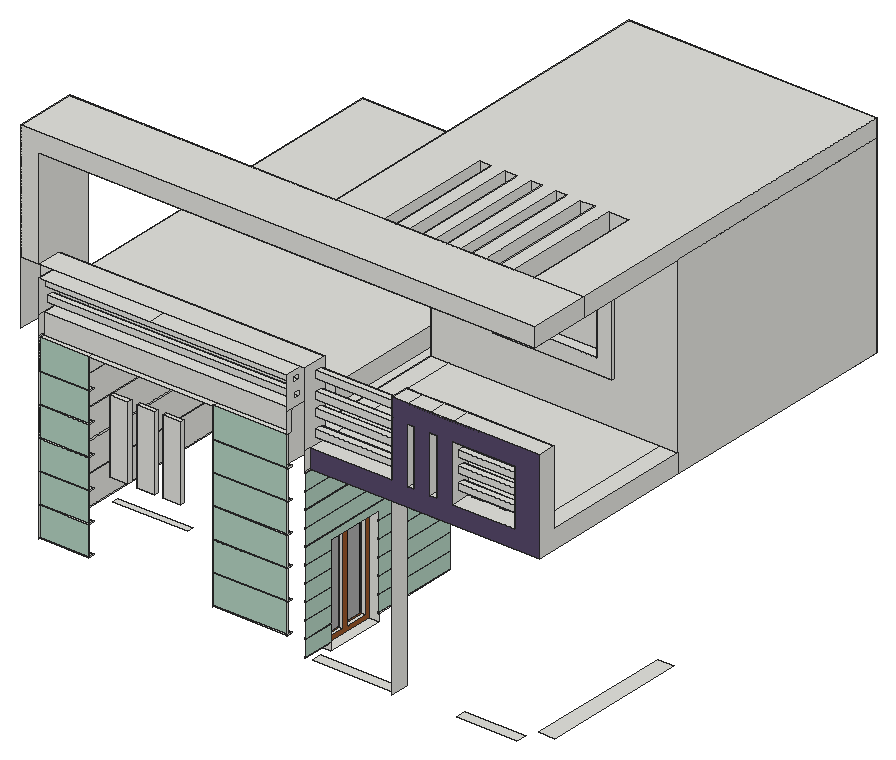
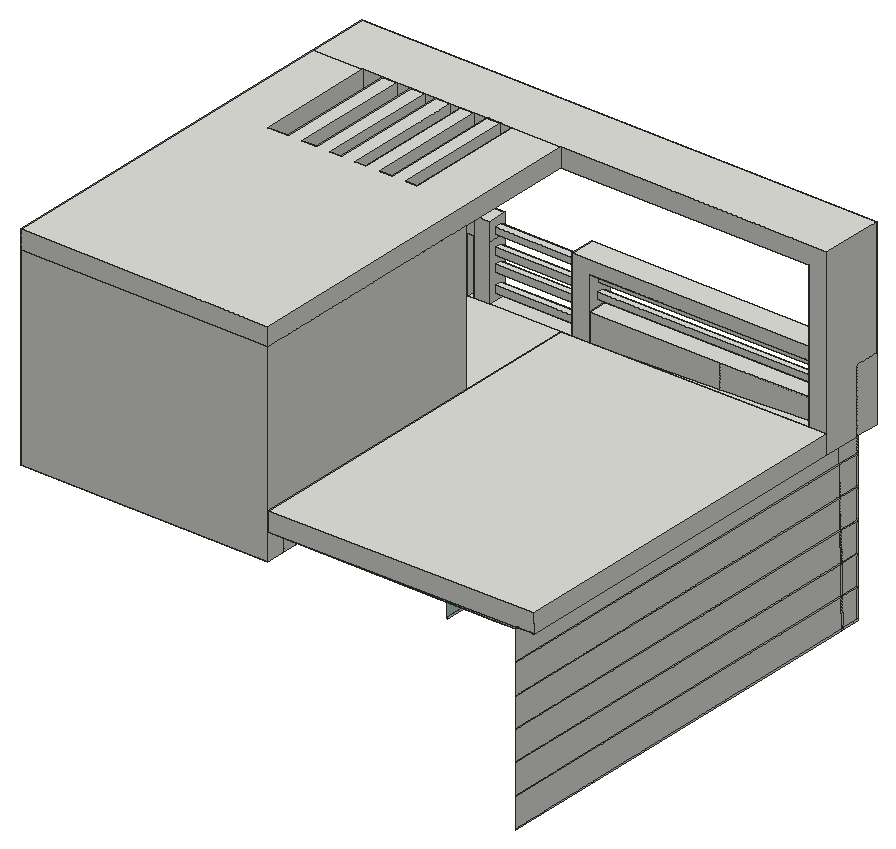
# SketchUp Ruby script. Lengths in inches.
U = 1.inch
M = Sketchup.active_model
def pt(a) = Geom::Point3d.new(a.map { |v| v * U })
def face(e, loops, mat)
  f = e.add_face(loops[0].map { |a| pt(a) })
  loops[1..].each { |l| e.add_face(l.map { |a| pt(a) }).erase! }
  f.material = f.back_material = mat if mat
  f
end
# faces: each face lists its corners as indices into pts; further lists are holes
def faces(e, pts, list, mat = nil) = list.each { |f| face(e, (f[0].is_a?(Array) ? f : [f]).map { |l| l.map { |i| pts[i] } }, mat) }
# xy, xz, yz: faces in a plane at the given z, y or x. An outline is a flat list of corners, or four numbers for a rectangle; further outlines are holes
def ring(l) = l.size == 4 ? [[l[0], l[1]], [l[2], l[1]], [l[2], l[3]], [l[0], l[3]]] : l.each_slice(2).to_a
def flat(e, list, mat, &to3) = list.each { |f| face(e, (f[0].is_a?(Array) ? f : [f]).map { |l| ring(l).map { |u, v| to3.(u, v) } }, mat) }
def xy(e, z, list, mat = nil) = flat(e, list, mat) { |x, y| [x, y, z] }
def xz(e, y, list, mat = nil) = flat(e, list, mat) { |x, z| [x, y, z] }
def yz(e, x, list, mat = nil) = flat(e, list, mat) { |y, z| [x, y, z] }
def lines(e, pts, list) = list.each { |a, b| e.add_line(pt(pts[a]), pt(pts[b])) }
# prism: a flat outline (further loops are holes) pulled along v
def prism(e, loops, v, mat = nil)
  f = face(e, loops, mat); d = Geom::Vector3d.new(v.map { |x| x * U })
  f.pushpull(f.normal.samedirection?(d) ? d.length : -d.length)
end
def box(e, o, s, mat = nil) = prism(e, [[o, [o[0] + s[0], o[1], o[2]], [o[0] + s[0], o[1] + s[1], o[2]], [o[0], o[1] + s[1], o[2]]]], [0, 0, s[2]], mat)
def at(x, y, z, deg = 0) = Geom::Transformation.translation(pt([x, y, z])) * Geom::Transformation.rotation(ORIGIN, Z_AXIS, deg.degrees)
def axes(o, x, y, z) = Geom::Transformation.new([*x, 0, *y, 0, *z, 0, *pt(o).to_a, 1])
def part(name) = M.definitions.add(name)
# library, detail: a bought-in or finely detailed component or shape, given as its bounding box
def library(name, o, s) = part(name).tap { |d| box(d.entities, o, s) }
def detail(e, o, s) = box(e.add_group.entities, o, s)
def put(e, d, t, mat = nil) = e.add_instance(d, t).tap { |i| i.material = mat if mat }
def group(e, t, mat = nil) = e.add_group.tap { |g| g.transformation = t; g.material = mat if mat }.entities
root = M.entities
M.materials.add("0235 AP 9121 dancing pink").color = [178, 209, 192]
M.materials.add("0259 AP 9618 Primrose Purple-N").color = [86, 72, 105]
M.materials.add("[0137_Black]").color = [17, 17, 17]
M.materials.add("[Translucent Glass Blue]").color = [0, 0, 0]
M.materials["[Translucent Glass Blue]"].alpha = 0.5
M.materials.add("[Wood Cherry Original]").color = [152, 86, 42]
c1 = part("Group\#4")
xy(c1.entities,0,[[0,0,2,29]])
xy(c1.entities,2,[[0,2,2,13.5],[0,15.5,2,27]])
xy(c1.entities,46,[[0,2,2,13.5],[0,15.5,2,27]])
xy(c1.entities,48,[[0,0,2,29]])
xz(c1.entities,0,[[0,0,2,48]],"[Wood Cherry Original]")
xz(c1.entities,2,[[0,2,2,46]])
xz(c1.entities,13.5,[[0,2,2,46]])
xz(c1.entities,15.5,[[0,2,2,46]])
xz(c1.entities,27,[[0,2,2,46]])
xz(c1.entities,29,[[0,0,2,48]])
yz(c1.entities,0,[[2,2,13.5,46],[15.5,2,27,46]],"[Translucent Glass Blue]")
yz(c1.entities,0,[[[0,0,29,48],[2,2,13.5,46],[15.5,2,27,46]]],"[Wood Cherry Original]")
yz(c1.entities,2,[[[0,0,29,48],[2,2,13.5,46],[15.5,2,27,46]]],"[Wood Cherry Original]")
c2 = part("Glass Door - Open Shower")
box(c2.entities,[0,0,0.95],[40,1.5,72])
xy(root,312,[[185.58,74.5,225.39,79.5],[255.27,74.5,284.65,79.5],[177,84.5,186.5,113.5],[287,84.5,295,156.5]])
xy(root,315.5,[[186,69.5,186.5,84.5],[186,113.5,186.5,156.5]])
xy(root,316,[[186,69.5,186.5,84.5],[186,113.5,186.5,156.5]])
xy(root,321.76,[[57,70,81,72.5],[141,70,177,72.5]])
xy(root,322.26,[[57,70,81,72.5],[141,70,177,72.5]])
xy(root,323.5,[[186,69.5,186.5,84.5],[186,113.5,186.5,156.5]])
xy(root,324,[[186,69.5,186.5,84.5],[186,113.5,186.5,156.5]])
xy(root,331.5,[[186,69.5,186.5,84.5],[186,113.5,186.5,156.5]])
xy(root,332,[[186,69.5,186.5,84.5],[186,113.5,186.5,156.5]])
xy(root,336.2,[[57,70,81,72.5],[141,70,177,72.5]])
xy(root,336.7,[[57,70,81,72.5],[141,70,177,72.5]])
xy(root,339.5,[[186,69.5,186.5,84.5],[186,113.5,186.5,156.5]])
xy(root,340,[[186,69.5,186.5,84.5],[186,113.5,186.5,156.5]])
xy(root,347.5,[[186,69.5,186.5,84.5],[186,113.5,186.5,156.5]])
xy(root,348,[[186,69.5,186.5,84.5],[186,113.5,186.5,156.5]])
xy(root,350.3125,[[93,69.5,129,72.5]])
xy(root,350.65,[[57,70,81,72.5],[141,70,177,72.5]])
xy(root,351.15,[[57,70,81,72.5],[141,70,177,72.5]])
xy(root,355.5,[[186,69.5,186.5,84.5],[186,113.5,186.5,156.5]])
xy(root,356,[[186,69.5,186.5,84.5],[186,113.5,186.5,156.5]])
xy(root,360,[[177,84.5,186.5,113.5],[193.71,156.5,229.71,165.5]])
xy(root,362.07,[[93,67.5,101.8125,69.5],[106,67.5,114.8125,69.5],[118.5625,67.5,127.375,69.5]])
xy(root,363.5,[[186,69.5,186.5,156.5]])
xy(root,364,[[186,69.5,186.5,156.5]])
xy(root,365.1,[[57,70,81,72.5],[141,70,177,72.5]])
xy(root,365.6,[[57,70,81,72.5],[141,70,177,72.5]])
xy(root,371.5,[[186,69.5,186.5,156.5]])
xy(root,372,[[186,69.5,186.5,156.5]])
xy(root,379.5,[[186,69.5,186.5,156.5]])
xy(root,379.54,[[57,70,81,72.5],[141,70,177,72.5]])
xy(root,380,[[186,69.5,186.5,156.5]])
xy(root,380.04,[[57,70,81,72.5],[141,70,177,72.5]])
xy(root,387.5,[[186,69.5,186.5,156.5]])
xy(root,388,[[186,69.5,186.5,156.5]])
xy(root,393.99,[[57,70,81,72.5],[141,70,177,72.5]])
xy(root,394.49,[[57,70,81,72.5],[141,70,177,72.5]])
xy(root,395.5,[[186,69.5,186.5,156.5]])
xy(root,396,[[186,72.5,186,156.5,297,156.5,297,84.5,285,84.5,285,72.5,255.27,72.5,255.27,81.5,247.45,81.5,247.45,72.5,244.15,72.5,244.15,81.5,236.33,81.5,236.33,72.5,233.21,72.5,233.21,81.5,225.39,81.5,225.39,72.5],[285,72.5,297,84.5],[[177,156.5,297,276.5],[186,165.5,288,267.5]]])
xy(root,397.89,[[93,67.5,101.8125,69.5],[106,67.5,114.8125,69.5],[118.5625,67.5,127.375,69.5]])
xy(root,405,[[186,72.5,225.39,81.5],[233.21,72.5,236.33,81.5],[244.15,72.5,247.45,81.5],[255.27,72.5,285,81.5],[177,81.5,186,156.5],
  [186,81.5,288,156.5],[288,81.5,297,156.5],[186,165.5,288,267.5]])
xy(root,408.87,[[186,75.37,225.39,78.74]])
xy(root,408.9375,[[81,69.5,141,72.5],[57,70,81,72.5],[141,70,177,72.5],[57,81.5,66,276.5],[66,267.22,177,276.5]])
xy(root,409.9375,[[48,81.22,57,81.22,57,99.17,56.93,99.17,56.93,81.5,48,81.5],[48,99.17,57,276.5]])
xy(root,410.1,[[255.27,75.16,285,78.35]])
xy(root,412.25,[[186,75.37,225.39,78.74]])
xy(root,413.29,[[255.27,75.16,285,78.35]])
xy(root,417.48,[[255.27,75.16,285,78.35]])
xy(root,417.87,[[186,75.37,225.39,78.74]])
xy(root,418.9375,[[57,72.5,177,81.5]])
xy(root,420.66,[[255.27,75.16,285,78.35]])
xy(root,421.25,[[186,75.37,225.39,78.74]])
xy(root,422.45,[[57,74.11,177,77.24]])
xy(root,424.41,[[255.27,75.16,285,78.35]])
xy(root,425.18,[[186,75.37,225.39,78.74]])
xy(root,425.57,[[57,74.11,177,77.24]])
xy(root,426.38,[[207.94,155.5,265.63,156.5]])
xy(root,427.6,[[255.27,75.16,285,78.35]])
xy(root,428.56,[[186,75.37,225.39,78.74]])
xy(root,429.81,[[57,73.03,177,76.96]])
xy(root,432,[[233.21,72.5,236.33,81.5],[244.15,72.5,247.45,81.5],[255.27,72.5,285,81.5]])
xy(root,432.74,[[57,73.03,177,76.96]])
xy(root,433.4375,[[215,155.5,258.58,165.5]])
xy(root,434.18,[[186,75.37,225.39,78.74]])
xy(root,435,[[57,69.5,111,81.5],[111,69.5,177,81.5]])
xy(root,437.56,[[186,75.37,225.39,78.74]])
xy(root,441,[[48,69.5,56.93,81.5],[56.93,69.5,57,81.5],[57,69.5,186,81.5],[225.39,72.5,233.21,81.5],[233.21,72.5,244.15,81.5],
  [244.15,72.5,255.27,81.5],[255.27,72.5,297,81.5]])
xy(root,459.08,[[215,155.5,258.58,165.5]])
xy(root,466.13,[[207.94,155.5,265.63,156.5]])
xy(root,489,[[56.93,69.5,56.93,99.17,177,99.17,177,156.5,186,156.5,186,69.5],[186,69.5,186,156.5,201,156.5,201,99.17,206.4,99.17,206.4,99.125,213,99.125,213,99.17,297,99.17,297,69.5],[206.4,99.125,213,99.17],[206.4,99.17,213,156.5],[219.09,99.17,225.6875,156.5],
  [230.96,99.17,237.5625,156.5],[242.96,99.17,249.5625,156.5],[256.65,99.17,263.25,156.5],[273,99.17,297,156.5],[177,156.5,186,156.5,186,267.5,288,267.5,288,165.5,186,165.5,186,156.5,297,156.5,297,276.5,177,276.5]])
xy(root,498,[[48,69.5,297,69.5,297,99.17,213,99.17,213,99.125,206.4,99.125,206.4,99.17,48,99.17],[206.4,99.125,213,99.17],[177,99.17,201,99.17,201,156.5,206.4,156.5,206.4,99.17,213,99.17,213,156.5,219.09,156.5,219.09,99.17,225.6875,99.17,225.6875,156.5,230.96,156.5,230.96,99.17,237.5625,99.17,237.5625,156.5,242.96,156.5,242.96,99.17,249.5625,99.17,249.5625,156.5,256.65,156.5,256.65,99.17,263.25,99.17,263.25,156.5,273,156.5,273,99.17,297,99.17,297,276.5,177,276.5]])
xz(root,67.5,[[93,362.07,101.8125,397.89],[106,362.07,114.8125,397.89],[118.5625,362.07,127.375,397.89]])
xz(root,69.5,[[48,441,56.93,441,56.93,489,297,489,297,498,48,498]])
xz(root,70,[[57,322.26,81,336.2],[141,322.26,177,336.2],[57,336.7,81,350.65],[141,336.7,177,350.65],[57,351.15,81,365.1],
  [141,351.15,177,365.1],[57,365.6,81,379.54],[141,365.6,177,379.54],[57,380.04,81,393.99],[141,380.04,177,393.99],
  [57,394.49,81,408.9375],[141,394.49,177,408.9375]],"0235 AP 9121 dancing pink")
xz(root,72.5,[[57,408.9375,177,418.9375]])
xz(root,72.5,[[186,396,297,396,297,441,225.39,441,225.39,432,285,432,285,405,255.27,405,255.27,432,247.45,432,247.45,405,244.15,405,244.15,432,236.33,432,236.33,405,233.21,405,233.21,432,225.39,432,225.39,405,186,405]],"0259 AP 9618 Primrose Purple-N")
xz(root,72.5,[[57,321.76,81,322.26],[141,321.76,177,322.26],[57,336.2,81,336.7],[141,336.2,177,336.7],[57,350.65,81,351.15],
  [141,350.65,177,351.15],[57,365.1,81,365.6],[141,365.1,177,365.6],[57,379.54,81,380.04],[141,379.54,177,380.04],
  [57,393.99,81,394.49],[141,393.99,177,394.49]],"[0137_Black]")
xz(root,73.03,[[57,429.81,177,432.74]])
xz(root,74.11,[[57,422.45,177,425.57]])
xz(root,75.16,[[255.27,410.1,285,413.29],[255.27,417.48,285,420.66],[255.27,424.41,285,427.6]])
xz(root,75.37,[[186,408.87,225.39,412.25],[186,417.87,225.39,421.25],[186,425.18,225.39,428.56],[186,434.18,225.39,437.56]])
xz(root,76.96,[[57,429.81,177,432.74]])
xz(root,77.24,[[57,422.45,177,425.57]])
xz(root,78.35,[[255.27,410.1,285,413.29],[255.27,417.48,285,420.66],[255.27,424.41,285,427.6]])
xz(root,78.74,[[186,408.87,225.39,412.25],[186,417.87,225.39,421.25],[186,425.18,225.39,428.56],[186,434.18,225.39,437.56]])
xz(root,81.5,[[177,405,177,435,57,435,57,441,186,441,186,405],[177,405,114,407.23,114,418.9375,177,418.9375],[225.39,405,233.21,441],[236.33,405,236.33,432,233.21,432,233.21,441,244.15,441,244.15,405],[247.45,405,247.45,432,244.15,432,244.15,441,255.27,441,255.27,405],
  [285,405,285,432,255.27,432,255.27,441,297,441,297,405],[114,407.23,66,408.9375,66,418.9375,114,418.9375],[57,408.9375,66,418.9375],[48,409.9375,56.93,418.9375],[48,418.9375,56.93,441],
  [56.93,418.9375,57,441]])
xz(root,84.5,[[177,312,177,360,186.5,360,186.5,356,186,356,186,355.5,186.5,355.5,186.5,348,186,348,186,347.5,186.5,347.5,186.5,340,186,340,186,339.5,186.5,339.5,186.5,332,186,332,186,331.5,186.5,331.5,186.5,324,186,324,186,323.5,186.5,323.5,186.5,316,186,316,186,315.5,186.5,315.5,186.5,312]])
xz(root,99.125,[[206.4,489,213,498]])
xz(root,99.17,[[177,408.9375,177,417.9375,56.93,418.87,56.93,409.9375,57,409.9375,57,409.87],[48,409.9375,48,498,177,498,177,489,56.93,489,56.93,418.87,48.07,418.9375],[48,409.9375,48.07,418.9375,56.93,418.87,56.93,409.9375],[201,489,219.09,498],[219.09,489,225.6875,498],
  [225.6875,489,230.96,498],[230.96,489,237.5625,498],[237.5625,489,242.96,498],[242.96,489,249.5625,498],[249.5625,489,256.65,498],
  [256.65,489,263.25,498],[263.25,489,273,498]])
xz(root,113.5,[[177,312,186.5,312,186.5,315.5,186,315.5,186,316,186.5,316,186.5,323.5,186,323.5,186,324,186.5,324,186.5,331.5,186,331.5,186,332,186.5,332,186.5,339.5,186,339.5,186,340,186.5,340,186.5,347.5,186,347.5,186,348,186.5,348,186.5,355.5,186,355.5,186,356,186.5,356,186.5,360,177,360]])
xz(root,155.5,[[[207.94,426.38,265.63,466.13],[215,433.4375,258.58,459.08]]])
xz(root,156.5,[[[177,405,297,489],[207.94,426.38,265.63,466.13]],[201,489,206.4,498],[213,489,219.09,498],[225.6875,489,230.96,498],[237.5625,489,242.96,498],
  [249.5625,489,256.65,498],[263.25,489,273,498]])
xz(root,165.5,[[[186,405,288,489],[215,433.4375,258.58,459.08]]])
xz(root,267.22,[[177,405,177,408.9375,66,408.9375]])
xz(root,267.5,[[186,405,288,489]])
xz(root,276.5,[[177,396,177,408.9375,177.07,417.9375,177,417.9375,177,489,297,489,297,396],[177,408.9375,57,409.87,57,409.9375,48,409.9375,48.07,418.9375,177,417.9375],[57,408.9375,57,409.87,177,408.9375],[177,408.9375,177,417.9375,177.07,417.9375],[57,409.87,48,409.9375,57,409.9375],
  [177,489,297,498]])
yz(root,48,[[69.5,409.9375,69.5,441,81.5,441,81.5,418.9375,81.22,409.9375],[81.5,409.9375,81.5,441,69.5,441,69.5,498,99.17,498,99.17,409.9375]])
yz(root,56.93,[[81.5,409.9375,99.17,409.9375,99.17,489,69.5,489,69.5,441,81.5,441]])
yz(root,57,[[69.5,321.76,72.5,322.26],[72.5,321.76,72.5,322.26,78.45,322.26,78.43,321.76],[78.43,321.76,79.41,321.76,79.42,322.26,78.45,322.26],[79.41,321.76,79.42,322.26,276.5,322.26,276.5,321.76],[69.5,322.26,70,336.2],
  [70,322.26,70,336.2,78.89,336.2,78.45,322.26],[78.45,322.26,79.42,322.26,79.72,336.2,78.89,336.2],[79.42,322.26,79.72,336.2,276.5,336.2,276.5,322.26],[69.5,336.2,72.5,336.7],[72.5,336.2,72.5,336.7,78.9,336.7,78.89,336.2],
  [78.89,336.2,79.72,336.2,79.73,336.7,78.9,336.7],[79.72,336.2,79.73,336.7,276.5,336.7,276.5,336.2],[69.5,336.7,70,350.65],[70,336.7,70,350.65,79.34,350.65,78.9,336.7],[78.9,336.7,79.73,336.7,80.03,350.65,79.34,350.65],
  [79.73,336.7,80.03,350.65,276.5,350.65,276.5,336.7],[69.5,350.65,72.5,351.15],[72.5,350.65,72.5,351.15,79.36,351.15,79.34,350.65],[79.34,350.65,80.03,350.65,80.04,351.15,79.36,351.15],[80.03,350.65,80.04,351.15,276.5,351.15,276.5,350.65],
  [69.5,351.15,70,365.1],[70,351.15,70,365.1,79.8,365.1,79.36,351.15],[79.36,351.15,80.04,351.15,80.34,365.1,79.8,365.1],[80.04,351.15,80.34,365.1,276.5,365.1,276.5,351.15],[69.5,365.1,72.5,365.6],
  [72.5,365.1,72.5,365.6,79.82,365.6,79.8,365.1],[79.8,365.1,80.34,365.1,80.35,365.6,79.82,365.6],[80.34,365.1,80.35,365.6,276.5,365.6,276.5,365.1],[69.5,365.6,70,379.54],[70,365.6,70,379.54,80.26,379.54,79.82,365.6],
  [79.82,365.6,80.35,365.6,80.65,379.54,80.26,379.54],[80.35,365.6,80.65,379.54,276.5,379.54,276.5,365.6],[69.5,379.54,72.5,380.04],[72.5,379.54,72.5,380.04,80.27,380.04,80.26,379.54],[80.26,379.54,80.65,379.54,80.66,380.04,80.27,380.04],
  [80.65,379.54,80.66,380.04,276.5,380.04,276.5,379.54],[69.5,380.04,70,393.99],[70,380.04,70,393.99,80.71,393.99,80.27,380.04],[80.27,380.04,80.66,380.04,80.96,393.99,80.71,393.99],[80.66,380.04,80.96,393.99,276.5,393.99,276.5,380.04],
  [69.5,393.99,72.5,394.49],[72.5,393.99,72.5,394.49,80.73,394.49,80.71,393.99],[80.71,393.99,80.96,393.99,80.97,394.49,80.73,394.49],[80.96,393.99,80.97,394.49,276.5,394.49,276.5,393.99],[69.5,394.49,70,408.9375],
  [70,394.49,70,408.9375,81.18,408.9375,80.73,394.49],[80.73,394.49,80.97,394.49,81.29,408.9375,81.18,408.9375],[80.97,394.49,81.29,408.9375,276.5,408.9375,276.5,394.49],[69.5,408.9375,72.5,409.9375],[72.5,408.9375,72.5,409.9375,81.22,409.9375,81.18,408.9375],
  [81.18,408.9375,81.29,408.9375,81.31,409.9375,81.22,409.9375],[81.29,408.9375,81.31,409.9375,81.5,409.9375,81.5,408.9375],[81.5,408.9375,276.5,408.9375,276.5,409.87,99.17,409.87,99.17,409.9375,81.5,409.9375],[99.17,409.87,276.5,409.9375],[69.5,409.9375,72.5,418.9375],
  [72.5,409.9375,72.5,418.9375,81.5,418.9375,81.22,409.9375],[81.31,409.9375,81.5,418.9375,81.5,409.9375],[[69.5,418.9375,81.5,435],[73.03,429.81,76.96,432.74],[74.11,422.45,77.24,425.57]]])
yz(root,81,[[69.5,321.76,72.5,322.26],[69.5,322.26,70,336.2],[69.5,336.2,72.5,336.7],[69.5,336.7,70,350.65],[69.5,350.65,72.5,351.15],
  [69.5,351.15,70,365.1],[69.5,365.1,72.5,365.6],[69.5,365.6,70,379.54],[69.5,379.54,72.5,380.04],[69.5,380.04,70,393.99],
  [69.5,393.99,72.5,394.49],[69.5,394.49,70,408.9375]])
yz(root,93,[[67.5,362.07,69.5,397.89]])
yz(root,101.8125,[[67.5,362.07,69.5,397.89]])
yz(root,106,[[67.5,362.07,69.5,397.89]])
yz(root,114.8125,[[67.5,362.07,69.5,397.89]])
yz(root,118.5625,[[67.5,362.07,69.5,397.89]])
yz(root,127.375,[[67.5,362.07,69.5,397.89]])
yz(root,141,[[69.5,321.76,72.5,322.26],[69.5,322.26,70,336.2],[69.5,336.2,72.5,336.7],[69.5,336.7,70,350.65],[69.5,350.65,72.5,351.15],
  [69.5,351.15,70,365.1],[69.5,365.1,72.5,365.6],[69.5,365.6,70,379.54],[69.5,379.54,72.5,380.04],[69.5,380.04,70,393.99],
  [69.5,393.99,72.5,394.49],[69.5,394.49,70,408.9375]])
yz(root,177,[[69.5,321.76,72.5,322.26],[69.5,322.26,70,336.2],[69.5,336.2,72.5,336.7],[69.5,336.7,70,350.65],[69.5,350.65,72.5,351.15],
  [69.5,351.15,70,365.1],[69.5,365.1,72.5,365.6],[69.5,365.6,70,379.54],[69.5,379.54,72.5,380.04],[69.5,380.04,70,393.99],
  [69.5,393.99,72.5,394.49],[69.5,394.49,70,396],[69.5,396,70,408.9375],[70,396,70,408.9375,72.5,408.9375,72.5,418.9375,81.5,418.9375,81.5,396],[81.5,396,267.22,405],
  [267.22,396,276.5,408.9375],[156.5,405,267.22,408.9375],[69.5,408.9375,72.5,418.9375],[99.17,408.9375,156.5,417.9375],[156.5,408.9375,276.5,417.9375],
  [156.5,417.9375,276.5,489],[[69.5,418.9375,81.5,435],[73.03,429.81,76.96,432.74],[74.11,422.45,77.24,425.57]],[99.17,489,276.5,498]])
yz(root,186,[[69.5,315.5,84.5,316],[113.5,315.5,156.5,316],[69.5,323.5,84.5,324],[113.5,323.5,156.5,324],[69.5,331.5,84.5,332],
  [113.5,331.5,156.5,332],[69.5,339.5,84.5,340],[113.5,339.5,156.5,340],[69.5,347.5,84.5,348],[113.5,347.5,156.5,348],
  [69.5,355.5,84.5,356],[113.5,355.5,156.5,356],[69.5,363.5,156.5,364],[69.5,371.5,156.5,372],[69.5,379.5,156.5,380],
  [69.5,387.5,156.5,388],[69.5,395.5,156.5,396],[69.5,396,72.5,405],[[69.5,405,81.5,441],[75.37,434.18,78.74,437.56],[75.37,425.18,78.74,428.56],[75.37,417.87,78.74,421.25],[75.37,408.87,78.74,412.25]],[165.5,405,267.5,489]])
yz(root,186.5,[[69.5,316,84.5,323.5],[113.5,316,156.5,323.5],[69.5,324,84.5,331.5],[113.5,324,156.5,331.5],[69.5,332,84.5,339.5],
  [113.5,332,156.5,339.5],[69.5,340,84.5,347.5],[113.5,340,156.5,347.5],[69.5,348,84.5,355.5],[113.5,348,156.5,355.5],
  [69.5,356,84.5,356,84.5,360,113.5,360,113.5,356,156.5,356,156.5,363.5,69.5,363.5],[69.5,364,156.5,371.5],[69.5,372,156.5,379.5],[69.5,380,156.5,387.5],[69.5,388,156.5,395.5]],"0235 AP 9121 dancing pink")
yz(root,201,[[99.17,489,156.5,498]])
yz(root,206.4,[[99.125,489,156.5,498]])
yz(root,207.94,[[155.5,426.38,156.5,466.13]])
yz(root,213,[[99.125,489,156.5,498]])
yz(root,215,[[155.5,433.4375,165.5,459.08]])
yz(root,219.09,[[99.17,489,156.5,498]])
yz(root,225.39,[[72.5,312,81.5,396],[[72.5,405,81.5,432],[75.37,425.18,78.74,428.56],[75.37,417.87,78.74,421.25],[75.37,408.87,78.74,412.25]],[[72.5,432,81.5,441],[75.37,434.18,78.74,437.56]]])
yz(root,225.6875,[[99.17,489,156.5,498]])
yz(root,230.96,[[99.17,489,156.5,498]])
yz(root,233.21,[[72.5,405,81.5,432]])
yz(root,236.33,[[72.5,405,81.5,432]])
yz(root,237.5625,[[99.17,489,156.5,498]])
yz(root,242.96,[[99.17,489,156.5,498]])
yz(root,244.15,[[72.5,405,81.5,432]])
yz(root,247.45,[[72.5,405,81.5,432]])
yz(root,249.5625,[[99.17,489,156.5,498]])
yz(root,255.27,[[[72.5,405,81.5,432],[75.16,424.41,78.35,427.6],[75.16,417.48,78.35,420.66],[75.16,410.1,78.35,413.29]]])
yz(root,256.65,[[99.17,489,156.5,498]])
yz(root,258.58,[[155.5,433.4375,165.5,459.08]])
yz(root,263.25,[[99.17,489,156.5,498]])
yz(root,265.63,[[155.5,426.38,156.5,466.13]])
yz(root,273,[[99.17,489,156.5,498]])
yz(root,285,[[[72.5,405,81.5,432],[75.16,424.41,78.35,427.6],[75.16,417.48,78.35,420.66],[75.16,410.1,78.35,413.29]]])
yz(root,288,[[165.5,405,267.5,489]])
yz(root,297,[[72.5,396,156.5,396,156.5,405,81.5,405,81.5,441,72.5,441],[156.5,396,276.5,489],[69.5,489,99.17,498],[99.17,489,276.5,498]])
p = [[66,81.5,408.9375],[114,81.5,407.23],[177,81.5,405],[177,156.5,405],[177,242.81,405],[66,242.81,408.9375],
  [66,267.22,408.9375],[177,267.22,405],[57,276.5,409.87],[177,276.5,408.9375],[177,267.22,408.9375],[177,156.5,408.9375],
  [177,99.17,408.9375],[57,99.17,409.87],[57,81.5,418.9375],[57,81.22,409.9375],[48,81.22,409.9375],[48,81.5,418.9375],
  [56.93,81.5,418.9375],[48.07,276.5,418.9375],[48,276.5,409.9375],[48,99.17,409.9375],[48.07,99.17,418.9375],[177,276.5,417.9375],
  [56.93,99.17,418.87],[177,99.17,417.9375],[177,156.5,417.9375],[186,165.5,405],[186,156.5,405]]
faces(root,p,[[0,1,2,3,4,5],[6,5,4,7],[8,9,10,11,12,13],[14,15,16,17,18],[19,20,21,22],[23,19,22,24,25,26]])
lines(root,p,[[27,28]])
put(root,c1,at(179.5,84.5,312))
put(root,c2,axes([215,160.5,433.36],[1.08935,0,0],[0,0.27223,0],[0,0,0.35245]))
